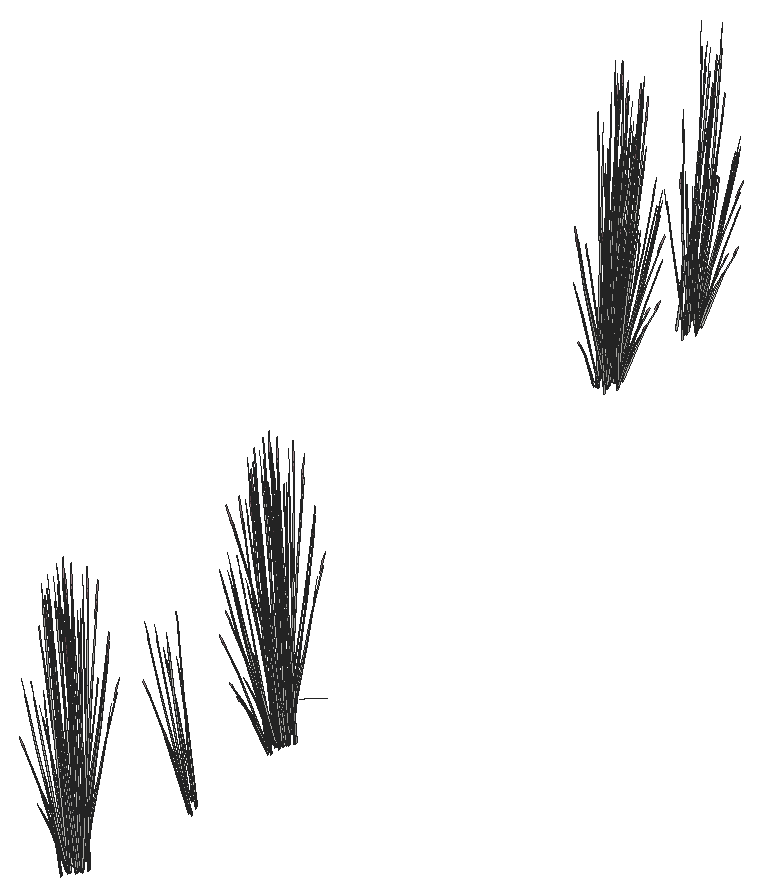
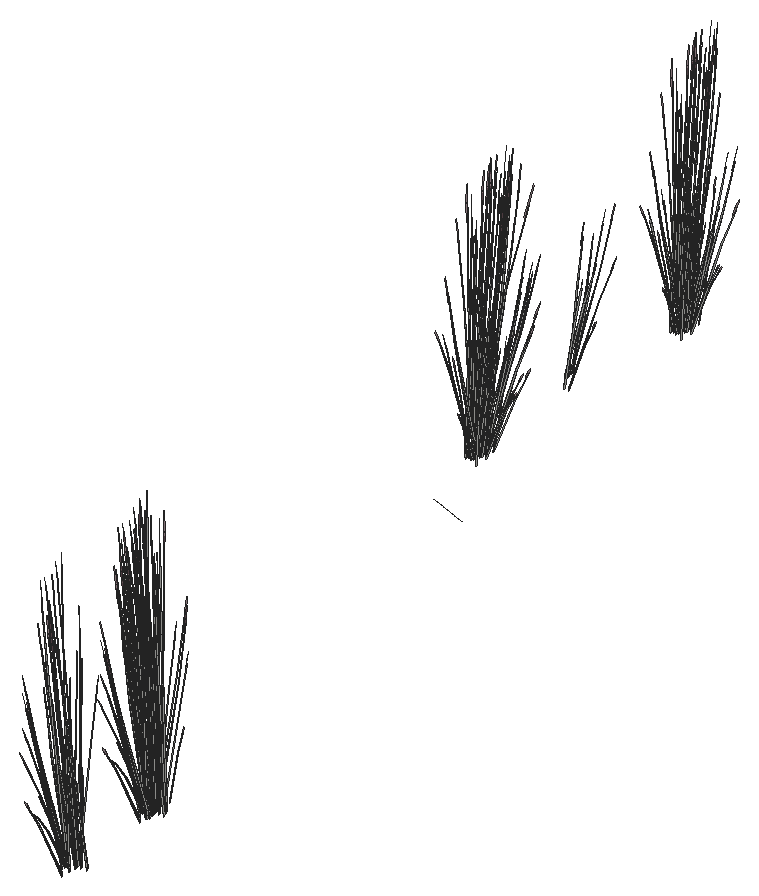
# SketchUp Ruby script. Lengths in inches.
U = 1.inch
M = Sketchup.active_model
def pt(a) = Geom::Point3d.new(a.map { |v| v * U })
def face(e, loops, mat)
  f = e.add_face(loops[0].map { |a| pt(a) })
  loops[1..].each { |l| e.add_face(l.map { |a| pt(a) }).erase! }
  f.material = f.back_material = mat if mat
  f
end
# faces: each face lists its corners as indices into pts; further lists are holes
def faces(e, pts, list, mat = nil) = list.each { |f| face(e, (f[0].is_a?(Array) ? f : [f]).map { |l| l.map { |i| pts[i] } }, mat) }
# xy, xz, yz: faces in a plane at the given z, y or x. An outline is a flat list of corners, or four numbers for a rectangle; further outlines are holes
def ring(l) = l.size == 4 ? [[l[0], l[1]], [l[2], l[1]], [l[2], l[3]], [l[0], l[3]]] : l.each_slice(2).to_a
def flat(e, list, mat, &to3) = list.each { |f| face(e, (f[0].is_a?(Array) ? f : [f]).map { |l| ring(l).map { |u, v| to3.(u, v) } }, mat) }
def xy(e, z, list, mat = nil) = flat(e, list, mat) { |x, y| [x, y, z] }
def xz(e, y, list, mat = nil) = flat(e, list, mat) { |x, z| [x, y, z] }
def yz(e, x, list, mat = nil) = flat(e, list, mat) { |y, z| [x, y, z] }
def lines(e, pts, list) = list.each { |a, b| e.add_line(pt(pts[a]), pt(pts[b])) }
# prism: a flat outline (further loops are holes) pulled along v
def prism(e, loops, v, mat = nil)
  f = face(e, loops, mat); d = Geom::Vector3d.new(v.map { |x| x * U })
  f.pushpull(f.normal.samedirection?(d) ? d.length : -d.length)
end
def box(e, o, s, mat = nil) = prism(e, [[o, [o[0] + s[0], o[1], o[2]], [o[0] + s[0], o[1] + s[1], o[2]], [o[0], o[1] + s[1], o[2]]]], [0, 0, s[2]], mat)
def at(x, y, z, deg = 0) = Geom::Transformation.translation(pt([x, y, z])) * Geom::Transformation.rotation(ORIGIN, Z_AXIS, deg.degrees)
def axes(o, x, y, z) = Geom::Transformation.new([*x, 0, *y, 0, *z, 0, *pt(o).to_a, 1])
def part(name) = M.definitions.add(name)
# library, detail: a bought-in or finely detailed component or shape, given as its bounding box
def library(name, o, s) = part(name).tap { |d| box(d.entities, o, s) }
def detail(e, o, s) = box(e.add_group.entities, o, s)
def put(e, d, t, mat = nil) = e.add_instance(d, t).tap { |i| i.material = mat if mat }
def group(e, t, mat = nil) = e.add_group.tap { |g| g.transformation = t; g.material = mat if mat }.entities
root = M.entities
M.materials.add("LightPink_Translucent").color = [144, 107, 117]
M.materials["LightPink_Translucent"].alpha = 0.75
c1 = part("blade")
p = [[2.15,0.21,22],[0,0.17,0],[0.09,0.45,0],[2.18,0.31,22],[2.29,0.31,22],[0.38,0.45,0],
  [2.48,0.24,33],[2.49,0.24,33],[2.48,0.22,33]]
faces(c1.entities,p,[[0,1,2,3],[4,5,2,3],[6,3,4,7],[8,0,3,6]])
c2 = part("seeds")
p = [[0.3,-0.1,1.38],[-0.01,-0.03,1.59],[-0.01,-0.03,0.03],[0.14,-0.07,-0.07],[0.29,-0.03,3],[0.15,0.01,3.11]]
faces(c2.entities,p,[[0,1,2,3],[1,0,4,5]],"LightPink_Translucent")
c3 = part("blade with seeds")
put(c3.entities,c1,at(0,0,0))
put(c3.entities,c2,axes([2.4,0.25,30.99],[1.5799,-0.05474,1.17369],[-0.12525,1.92788,0.29478],[-0.07173,-0.02425,1.56792]))
p = [[428.41,225.85,0],[423,225.85,-2]]
lines(root,p,[[0,1]])
put(root,c3,axes([402.14,327.82,-0.11],[-0.47029,-0.00441,-0.0428],[0,-0.61671,0.42951],[-0.01478,0.14039,1.36183]))
put(root,c3,axes([401.22,325.96,0.13],[-0.40434,0.14646,0.15172],[-0.09984,-0.54504,0.30174],[0.03606,0.07941,1.3795]))
put(root,c3,axes([399.88,348.72,-0.12],[0.39505,-0.18722,-0.1651],[0.13882,0.53931,0.00007],[0.04361,-0.02069,1.49552]))
put(root,c3,axes([400.8,323.92,0.38],[0.04827,0.32177,0.9878],[-0.26778,-0.17821,0.72577],[0.02882,-0.16476,0.21757]))
put(root,c3,axes([400.56,326.76,0.03],[-0.312,0.50076,0.39349],[-0.37066,-0.44204,0.15441],[0.07522,-0.04998,1.36617]))
put(root,c3,axes([401.09,327.55,-0.1],[0.26266,0.35642,0],[-0.26266,0.35642,0],[0,0,1.45569]))
put(root,c3,axes([401.08,327.13,0.34],[0.18257,-0.49721,0.38476],[0.37935,0.23929,-0.18517],[0,0.11462,1.23533]))
put(root,c3,axes([400.93,328.86,-0.1],[0.37935,0.24773,0],[-0.18257,0.51475,0],[0,0,1.5046]))
put(root,c3,axes([399.89,347.11,-0.1],[0.22605,0.46315,-0.38476],[-0.34239,0.32614,0.18517],[0.07315,0.05731,1.23533]))
put(root,c3,axes([400.39,329.51,2.03],[0.3699,0.13833,-0.43945],[-0.12679,0.47426,-0.34039],[0.03392,0.19095,0.84085]))
put(root,c3,axes([400.47,345.48,1.89],[0.2546,-0.29052,-0.30456],[0.24101,0.33173,0.39319],[0.03667,-0.16855,0.75234]))
put(root,c3,axes([400.96,327.01,0.05],[-0.4756,-0.11626,0.42311],[0.09679,-0.6566,0.16603],[0.0695,0.0634,1.46899]))
put(root,c3,axes([402.04,327.91,-0.26],[-0.26266,0.34428,-0.26641],[-0.26266,-0.34428,0.26641],[0,0.11089,1.19518]))
put(root,c3,axes([400.53,349.22,0.38],[-0.21187,-0.15866,0.9878],[0.27357,-0.16121,0.72577],[0.07379,0.13656,0.21757]))
put(root,c3,axes([399.77,349.05,0.23],[0.00664,-0.18292,1.22981],[0.31732,-0.20432,-0.26449],[0.09796,0.21893,0.52581]))
put(root,c3,axes([399.39,346.45,-0.23],[0.25345,-0.41475,-0.53624],[0.31485,0.37608,-0.14074],[0.10156,-0.10346,1.18365]))
put(root,c3,axes([401.29,327.84,-0.2],[0.13798,0.50522,-0.59522],[-0.39745,0.18195,-0.15622],[0.01525,0.17108,1.31385]))
put(root,c3,axes([401.1,327.3,-0.1],[0.42099,0,0],[0,0.57126,0],[0,0,1.5343]))
put(root,c3,axes([400.69,326.67,0.34],[-0.22605,-0.46315,0.38476],[0.34239,-0.32614,-0.18517],[0.07315,0.05731,1.23533]))
put(root,c3,axes([400.28,326.78,0.29],[-0.04385,-0.62963,-0.25022],[0.45669,-0.03807,-0.43002],[0.08042,-0.08387,1.37348]))
put(root,c3,axes([401.24,327.24,0.25],[0.35059,-0.16092,0.12452],[0.12277,0.45952,-0.35559],[0,0.10113,1.09]))
put(root,c3,axes([401.375,325.47,2.03],[-0.26937,-0.37076,-0.43945],[0.28456,-0.3247,-0.34039],[0.04099,-0.18838,0.84085]))
put(root,c3,axes([400.51,346.09,-0.26],[0.08839,0.48081,-0.26641],[-0.35106,0.13653,0.26641],[0.07077,0.05545,1.19518]))
put(root,c3,axes([401.17,347.65,0.04],[0.47052,0,0],[0,0.61671,-0.44382],[0,0.14046,1.40792]))
put(root,c3,axes([401.125,327.28,0.29],[0.42377,0.26329,-0.25022],[-0.20405,0.55571,-0.43002],[0.01332,0.13644,1.37348]))
put(root,c3,axes([399.65,346.85,0.29],[0.37992,-0.36634,-0.25022],[0.25264,0.51764,-0.43002],[0.09374,0.05257,1.37348]))
put(root,c3,axes([400.5625,349.9375,0.29],[-0.2413,-0.01731,0.90352],[0.15935,-0.36755,0.49885],[0.09532,0.13058,0.70873]))
put(root,c3,axes([400.22,325.39,-0.26],[0.35106,0.13653,-0.26641],[-0.08839,0.48081,0.26641],[0.07077,-0.05545,1.19518]))
put(root,c3,axes([401.2,324.81,0.23],[-0.10696,0.11169,1.22981],[-0.32033,-0.19549,-0.26449],[0.05938,-0.24312,0.52581]))
put(root,c3,axes([402.04,327.41,0.13],[0,-0.5518,0.427],[0.42099,0,0],[0,0.12568,1.35453]))
put(root,c3,axes([402.22,327.92,-0.26],[0,0.5518,-0.427],[-0.42099,0,0],[0,0.12568,1.35453]))
put(root,c3,axes([400.14,325.17,-0.26],[0.35217,-0.2759,-0.427],[0.2105,0.49473,0],[0.08021,-0.06284,1.35453]))
put(root,c3,axes([400.84,326.54,0.25],[0.07259,-0.49245,0.12452],[0.35466,0.08548,-0.35559],[0.06454,0.05057,1.09]))
put(root,c3,axes([398.6875,346.53,-0.63],[-0.37038,0.22092,1.10879],[-0.11789,-0.63387,0.43083],[0.22743,0.01055,1.26112]))
put(root,c3,axes([401.35,325.68,0.13],[-0.35217,-0.2759,0.427],[0.2105,-0.49473,0],[0.08021,0.06284,1.35453]))
put(root,c3,axes([401.46,325.64,2.28],[0.00979,-0.51041,-0.61099],[0.4123,0.03428,0.07373],[0.04351,-0.21623,0.8643]))
put(root,c3,axes([400.05,349.43,2.03],[0.37131,-0.13117,-0.43945],[0.06495,0.49674,-0.34039],[0.09973,0.14235,0.84085]))
put(root,c3,axes([401.04,328.5625,-0.12],[0.39505,-0.18722,-0.1651],[0.13882,0.53931,0.00007],[0.04361,-0.02069,1.49552]))
put(root,c3,axes([400.39,345.55,0.04],[0.23526,-0.55293,0],[0.3936,0.30836,-0.44382],[0.08964,0.07023,1.40792]))
put(root,c3,axes([400.78,345.31,-0.72],[-0.05632,-0.04347,1.51654],[-0.14467,-0.48565,-0.23168],[0.09759,-0.13179,0.25832]))
put(root,c3,axes([400.6,345.88,-0.26],[0.35217,0.2759,-0.427],[-0.2105,0.49473,0],[0.08021,0.06284,1.35453]))
put(root,c3,axes([400.59,349.8,-0.72],[0.02741,-0.07966,1.51654],[0.34514,-0.23462,-0.23168],[0.10464,0.12143,0.25832]))
put(root,c3,axes([400.77,346.47,2.03],[-0.09666,-0.50384,-0.43945],[0.36608,-0.08814,-0.34039],[0.10491,-0.13533,0.84085]))
put(root,c3,axes([401.05,326.96,-0.1],[0.22605,0.46315,-0.38476],[-0.34239,0.32614,0.18517],[0.07315,0.05731,1.23533]))
put(root,c3,axes([401.63,325.33,1.89],[0.2546,-0.29052,-0.30456],[0.24101,0.33173,0.39319],[0.03667,-0.16855,0.75234]))
put(root,c3,axes([400.09,346.9375,-0.23],[0.39143,0.09047,-0.53624],[-0.0826,0.55804,-0.14074],[0.11681,0.06762,1.18365]))
put(root,c3,axes([401.6875,329.0625,0.38],[-0.21187,-0.15866,0.9878],[0.27357,-0.16121,0.72577],[0.07379,0.13656,0.21757]))
put(root,c3,axes([400.94,328.89,0.23],[0.00664,-0.18292,1.22981],[0.31732,-0.20432,-0.26449],[0.09796,0.21893,0.52581]))
put(root,c3,axes([401.76,347.26,-0.06],[-0.23329,-0.35284,-0.05579],[0.2555,-0.3233,-0.25298],[0.0724,-0.02276,0.83441]))
put(root,c3,axes([400.56,326.3,-0.23],[0.25345,-0.41475,-0.53624],[0.31485,0.37608,-0.14074],[0.10156,-0.10346,1.18365]))
put(root,c3,axes([401.22,345.47,0.38],[-0.12533,0.28089,0.9878],[-0.10773,-0.37739,0.72577],[0.10352,-0.09457,0.21757]))
put(root,c3,axes([401.67,325.93,-0.26],[0.08839,0.48081,-0.26641],[-0.35106,0.13653,0.26641],[0.07077,0.05545,1.19518]))
put(root,c3,axes([402.33,327.5,0.04],[0.47052,0,0],[0,0.61671,-0.44382],[0,0.14046,1.40792]))
put(root,c3,axes([400.81,326.7,0.29],[0.37992,-0.36634,-0.25022],[0.25264,0.51764,-0.43002],[0.09374,0.05257,1.37348]))
put(root,c3,axes([401.72,329.78,0.29],[-0.2413,-0.01731,0.90352],[0.15935,-0.36755,0.49885],[0.09532,0.13058,0.70873]))
put(root,c3,axes([401.04,346.52,1.89],[0.32754,-0.07886,-0.30456],[0.08649,0.45081,0.39319],[0.09386,-0.12109,0.75234]))
put(root,c3,axes([400.78,346.68,2.28],[0.19655,-0.43539,-0.61099],[0.34443,0.30942,0.07373],[0.11736,-0.15774,0.8643]))
put(root,c3,axes([400.78,349.02,1.89],[0.2141,0.34548,-0.30456],[-0.24447,0.32704,0.39319],[0.12421,0.04976,0.75234]))
put(root,c3,axes([399.85,326.375,-0.63],[-0.37038,0.22092,1.10879],[-0.11789,-0.63387,0.43083],[0.22743,0.01055,1.26112]))
put(root,c3,axes([401.21,329.28,2.03],[0.37131,-0.13117,-0.43945],[0.06495,0.49674,-0.34039],[0.09973,0.14235,0.84085]))
put(root,c3,axes([401.55,325.39,0.04],[0.23526,-0.55293,0],[0.3936,0.30836,-0.44382],[0.08964,0.07023,1.40792]))
put(root,c3,axes([401.95,325.15,-0.72],[-0.05632,-0.04347,1.51654],[-0.14467,-0.48565,-0.23168],[0.09759,-0.13179,0.25832]))
put(root,c3,axes([401.77,325.73,-0.26],[0.35217,0.2759,-0.427],[-0.2105,0.49473,0],[0.08021,0.06284,1.35453]))
put(root,c3,axes([400.94,347.59,2.03],[0.10194,-0.50193,-0.43945],[0.34951,0.17204,-0.34039],[0.14072,-0.04602,0.84085]))
put(root,c3,axes([401.82,347.91,0.38],[-0.23249,0.0911,0.9878],[0.10944,-0.37648,0.72577],[0.12334,0.02576,0.21757]))
put(root,c3,axes([401.75,329.65,-0.72],[0.02741,-0.07966,1.51654],[0.34514,-0.23462,-0.23168],[0.10464,0.12143,0.25832]))
put(root,c3,axes([401.93,326.32,2.03],[-0.09666,-0.50384,-0.43945],[0.36608,-0.08814,-0.34039],[0.10491,-0.13533,0.84085]))
put(root,c3,axes([401.07,346.27,0.23],[-0.13443,-0.01634,1.22981],[-0.13772,-0.43844,-0.26449],[0.16514,-0.12403,0.52581]))
put(root,c3,axes([401.16,347.82,1.89],[0.31272,0.15393,-0.30456],[-0.09121,0.44909,0.39319],[0.1259,-0.04118,0.75234]))
put(root,c3,axes([401.25,326.78,-0.23],[0.39143,0.09047,-0.53624],[-0.0826,0.55804,-0.14074],[0.11681,0.06762,1.18365]))
put(root,c3,axes([402.92,327.11,-0.06],[-0.23329,-0.35284,-0.05579],[0.2555,-0.3233,-0.25298],[0.0724,-0.02276,0.83441]))
put(root,c3,axes([400.55,348.79,2.28],[0.37615,0.01329,-0.61099],[-0.02526,0.55946,0.07373],[0.15935,0.05904,0.8643]))
put(root,c3,axes([401.32,347.73,-0.3],[-0.24235,0.06622,1.21762],[-0.03858,-0.5271,0.0697],[0.16974,-0.07978,0.69287]))
put(root,c3,axes([402.38,325.32,0.38],[-0.12533,0.28089,0.9878],[-0.10773,-0.37739,0.72577],[0.10352,-0.09457,0.21757]))
put(root,c3,axes([401.58,347.39,-0.72],[-0.01967,-0.08377,1.51654],[0.1364,-0.49004,-0.23168],[0.13759,-0.00705,0.25832]))
put(root,c3,axes([400.875,347.77,2.28],[0.33065,-0.2437,-0.61099],[0.18427,0.50165,0.07373],[0.15976,-0.05699,0.8643]))
put(root,c3,axes([402.2,326.37,1.89],[0.32754,-0.07886,-0.30456],[0.08649,0.45081,0.39319],[0.09386,-0.12109,0.75234]))
put(root,c3,axes([401.94,326.52,2.28],[0.19655,-0.43539,-0.61099],[0.34443,0.30942,0.07373],[0.11736,-0.15774,0.8643]))
put(root,c3,axes([401.94,328.87,1.89],[0.2141,0.34548,-0.30456],[-0.24447,0.32704,0.39319],[0.12421,0.04976,0.75234]))
put(root,c3,axes([401.38,348.51,0.23],[-0.09062,-0.13571,1.22981],[0.11791,-0.44895,-0.26449],[0.18335,0.06082,0.52581]))
put(root,c3,axes([402.1,327.4375,2.03],[0.10194,-0.50193,-0.43945],[0.34951,0.17204,-0.34039],[0.14072,-0.04602,0.84085]))
put(root,c3,axes([402.98,327.76,0.38],[-0.23249,0.0911,0.9878],[0.10944,-0.37648,0.72577],[0.12334,0.02576,0.21757]))
put(root,c3,axes([402.23,326.12,0.23],[-0.13443,-0.01634,1.22981],[-0.13772,-0.43844,-0.26449],[0.16514,-0.12403,0.52581]))
put(root,c3,axes([402.32,327.67,1.89],[0.31272,0.15393,-0.30456],[-0.09121,0.44909,0.39319],[0.1259,-0.04118,0.75234]))
put(root,c3,axes([401.71,328.64,2.28],[0.37615,0.01329,-0.61099],[-0.02526,0.55946,0.07373],[0.15935,0.05904,0.8643]))
put(root,c3,axes([402.48,327.58,-0.3],[-0.24235,0.06622,1.21762],[-0.03858,-0.5271,0.0697],[0.16974,-0.07978,0.69287]))
put(root,c3,axes([402.74,327.23,-0.72],[-0.01967,-0.08377,1.51654],[0.1364,-0.49004,-0.23168],[0.13759,-0.00705,0.25832]))
put(root,c3,axes([402.04,327.62,2.28],[0.33065,-0.2437,-0.61099],[0.18427,0.50165,0.07373],[0.15976,-0.05699,0.8643]))
put(root,c3,axes([402.55,328.36,0.23],[-0.09062,-0.13571,1.22981],[0.11791,-0.44895,-0.26449],[0.18335,0.06082,0.52581]))
put(root,c3,axes([430.46,162.27,0.23],[0.13077,0.0453,1.22981],[0.08428,0.46268,-0.26449],[-0.17763,0.08661,0.52581]))
put(root,c3,axes([430.46,211.47,0.23],[0.13077,0.0453,1.22981],[0.08428,0.46268,-0.26449],[-0.17763,0.08661,0.52581]))
put(root,c3,axes([431.62,160.79,0.875],[0.10696,-0.07982,1.52275],[0.03688,0.55733,0.11917],[-0.23167,0.07395,0.54424]))
put(root,c3,axes([431.62,209.99,0.875],[0.10696,-0.07982,1.52275],[0.03688,0.55733,0.11917],[-0.23167,0.07395,0.54424]))
put(root,c3,axes([431.27,159.9,2.28],[-0.37615,-0.01329,-0.61099],[0.02526,-0.55946,0.07373],[-0.15935,-0.05904,0.8643]))
put(root,c3,axes([431.27,209.09,2.28],[-0.37615,-0.01329,-0.61099],[0.02526,-0.55946,0.07373],[-0.15935,-0.05904,0.8643]))
put(root,c3,axes([430.97,160.03,0.23],[0.07347,0.15363,1.22981],[-0.16929,0.41759,-0.26449],[-0.17383,-0.09981,0.52581]))
put(root,c3,axes([430.97,209.23,0.23],[0.07347,0.15363,1.22981],[-0.16929,0.41759,-0.26449],[-0.17383,-0.09981,0.52581]))
put(root,c3,axes([430.67,160.87,1.89],[-0.31272,-0.15393,-0.30456],[0.09121,-0.44909,0.39319],[-0.1259,0.04118,0.75234]))
put(root,c3,axes([430.88,161.1,2.03],[-0.10194,0.50193,-0.43945],[-0.34951,-0.17204,-0.34039],[-0.14072,0.04602,0.84085]))
put(root,c3,axes([430.88,210.29,2.03],[-0.10194,0.50193,-0.43945],[-0.34951,-0.17204,-0.34039],[-0.14072,0.04602,0.84085]))
put(root,c3,axes([431.15,160.01,2.03],[-0.27323,0.36552,-0.43945],[-0.23929,-0.38612,-0.34039],[-0.13882,-0.05561,0.84085]))
put(root,c3,axes([431.15,209.21,2.03],[-0.27323,0.36552,-0.43945],[-0.23929,-0.38612,-0.34039],[-0.13882,-0.05561,0.84085]))
put(root,c3,axes([430.71,161.06,-0.72],[0.00954,0.08696,1.51654],[-0.19238,0.45414,-0.23168],[-0.13665,-0.02289,0.25832]))
put(root,c3,axes([430.71,210.26,-0.72],[0.00954,0.08696,1.51654],[-0.19238,0.45414,-0.23168],[-0.13665,-0.02289,0.25832]))
put(root,c3,axes([430.19,163.24,0.38],[0.15682,-0.25009,0.9878],[0.06188,0.39591,0.72577],[-0.11333,0.07089,0.21757]))
put(root,c3,axes([430.19,212.4375,0.38],[0.15682,-0.25009,0.9878],[0.06188,0.39591,0.72577],[-0.11333,0.07089,0.21757]))
put(root,c3,axes([430.78,162.16,1.89],[-0.32754,0.07886,-0.30456],[-0.08649,-0.45081,0.39319],[-0.09386,0.12109,0.75234]))
put(root,c3,axes([430.6,163.5,-0.72],[0.05047,0.05513,1.51654],[0.08558,0.51079,-0.23168],[-0.11187,0.10892,0.25832]))
put(root,c3,axes([430.6,212.7,-0.72],[0.05047,0.05513,1.51654],[0.08558,0.51079,-0.23168],[-0.11187,0.10892,0.25832]))
put(root,c3,axes([430.53,160.5,0.38],[0.24023,-0.03948,0.9878],[-0.15239,0.3479,0.72577],[-0.11872,-0.05219,0.21757]))
put(root,c3,axes([430.53,209.69,0.38],[0.24023,-0.03948,0.9878],[-0.15239,0.3479,0.72577],[-0.11872,-0.05219,0.21757]))
put(root,c3,axes([431.05,162.21,2.03],[0.09666,0.50384,-0.43945],[-0.36608,0.08814,-0.34039],[-0.10491,0.13533,0.84085]))
put(root,c3,axes([431.05,211.41,2.03],[0.09666,0.50384,-0.43945],[-0.36608,0.08814,-0.34039],[-0.10491,0.13533,0.84085]))
put(root,c3,axes([431.97,161.85,-0.23],[-0.39143,-0.09047,-0.53624],[0.0826,-0.55804,-0.14074],[-0.11681,-0.06762,1.18365]))
put(root,c3,axes([431.97,211.05,-0.23],[-0.39143,-0.09047,-0.53624],[0.0826,-0.55804,-0.14074],[-0.11681,-0.06762,1.18365]))
put(root,c3,axes([431.93,208.43,2.28],[-0.32086,-0.26671,-0.61099],[0.22803,-0.46737,0.07373],[-0.11625,-0.15925,0.8643]))
put(root,c3,axes([431.78,208.45,2.03],[-0.37131,0.13117,-0.43945],[-0.06495,-0.49674,-0.34039],[-0.09973,-0.14235,0.84085]))
put(root,c3,axes([431.45,162.91,-0.26],[-0.35217,-0.2759,-0.427],[0.2105,-0.49473,0],[-0.08021,-0.06284,1.35453]))
put(root,c3,axes([431.45,212.11,-0.26],[-0.35217,-0.2759,-0.427],[0.2105,-0.49473,0],[-0.08021,-0.06284,1.35453]))
put(root,c3,axes([431.3,208,-0.72],[-0.03645,0.07269,1.51654],[-0.36835,0.15672,-0.23168],[-0.08898,-0.14257,0.25832]))
put(root,c3,axes([431.67,163.24,0.04],[-0.23526,0.55293,0],[-0.3936,-0.30836,-0.44382],[-0.08964,-0.07023,1.40792]))
put(root,c3,axes([431.67,212.4375,0.04],[-0.23526,0.55293,0],[-0.3936,-0.30836,-0.44382],[-0.08964,-0.07023,1.40792]))
put(root,c3,axes([431.24,164.04,0.23],[0.11874,-0.08705,1.22981],[0.29317,0.26247,-0.26449],[-0.08726,0.22711,0.52581]))
put(root,c3,axes([431.24,213.24,0.23],[0.11874,-0.08705,1.22981],[0.29317,0.26247,-0.26449],[-0.08726,0.22711,0.52581]))
put(root,c3,axes([431.07,159.08,-0.17],[-0.10855,0.45057,-0.03348],[-0.33409,-0.1386,-0.15179],[-0.05073,-0.0737,0.50065]))
put(root,c3,axes([431.07,208.28,-0.17],[-0.10855,0.45057,-0.03348],[-0.33409,-0.1386,-0.15179],[-0.05073,-0.0737,0.50065]))
put(root,c3,axes([431.57,207.71,0.23],[-0.02279,0.18051,1.22981],[-0.33311,0.15111,-0.26449],[-0.07787,-0.23331,0.52581]))
put(root,c3,axes([432.41,161.94,0.29],[-0.37992,0.36634,-0.25022],[-0.25264,-0.51764,-0.43002],[-0.09374,-0.05257,1.37348]))
put(root,c3,axes([432.41,211.13,0.29],[-0.37992,0.36634,-0.25022],[-0.25264,-0.51764,-0.43002],[-0.09374,-0.05257,1.37348]))
put(root,c3,axes([430.89,161.14,0.04],[-0.47052,0,0],[0,-0.61671,-0.44382],[0,-0.14046,1.40792]))
put(root,c3,axes([430.89,210.33,0.04],[-0.47052,0,0],[0,-0.61671,-0.44382],[0,-0.14046,1.40792]))
put(root,c3,axes([431.55,162.7,-0.26],[-0.08839,-0.48081,-0.26641],[0.35106,-0.13653,0.26641],[-0.07077,-0.05545,1.19518]))
put(root,c3,axes([431.55,211.9,-0.26],[-0.08839,-0.48081,-0.26641],[0.35106,-0.13653,0.26641],[-0.07077,-0.05545,1.19518]))
put(root,c3,axes([431.36,163.21,1.89],[-0.2546,0.29052,-0.30456],[-0.24101,-0.33173,0.39319],[-0.03667,0.16855,0.75234]))
put(root,c3,axes([432.66,162.34,-0.23],[-0.25345,0.41475,-0.53624],[-0.31485,-0.37608,-0.14074],[-0.10156,0.10346,1.18365]))
put(root,c3,axes([432.66,211.53,-0.23],[-0.25345,0.41475,-0.53624],[-0.31485,-0.37608,-0.14074],[-0.10156,0.10346,1.18365]))
put(root,c3,axes([431.25,160.97,0],[-0.35001,0.46392,0.2645],[-0.35022,-0.45904,-0.31383],[-0.01222,-0.13174,1.41801]))
put(root,c3,axes([431.25,210.17,0],[-0.35001,0.46392,0.2645],[-0.35022,-0.45904,-0.31383],[-0.01222,-0.13174,1.41801]))
put(root,c3,axes([432.69,211.45,0.86],[0.32517,0.22251,1.30084],[-0.31856,0.47936,0.51441],[-0.14269,-0.28411,1.09053]))
put(root,c3,axes([431.45,207.42,0.38],[0.19628,0.19205,0.9878],[-0.28586,0.11545,0.72577],[-0.06116,-0.1476,0.21757]))
put(root,c3,axes([432.84,162.1,0.12],[-0.36743,-0.44413,-0.21665],[0.30918,-0.49872,0.47412],[-0.09894,0.05195,1.44665]))
put(root,c3,axes([432.84,211.3,0.12],[-0.36743,-0.44413,-0.21665],[0.30918,-0.49872,0.47412],[-0.09894,0.05195,1.44665]))
put(root,c3,axes([432.17,161.68,-0.1],[-0.22605,-0.46315,-0.38476],[0.34239,-0.32614,0.18517],[-0.07315,-0.05731,1.23533]))
put(root,c3,axes([432.17,210.87,-0.1],[-0.22605,-0.46315,-0.38476],[0.34239,-0.32614,0.18517],[-0.07315,-0.05731,1.23533]))
put(root,c3,axes([431.53,162.9,2.59],[-0.00979,0.51041,-0.6782],[-0.4123,-0.03428,0.08184],[-0.04351,0.21623,0.95938]))
put(root,c3,axes([431.53,212.09,2.59],[-0.00979,0.51041,-0.6782],[-0.4123,-0.03428,0.08184],[-0.04351,0.21623,0.95938]))
put(root,c3,axes([431.52,164.33,0.38],[-0.00974,-0.3281,0.9878],[0.24334,0.23402,0.72577],[-0.04786,0.15639,0.21757]))
put(root,c3,axes([431.52,213.53,0.38],[-0.00974,-0.3281,0.9878],[0.24334,0.23402,0.72577],[-0.04786,0.15639,0.21757]))
put(root,c3,axes([432.65,162.01,-0.1],[-0.40861,0.03406,-0.38476],[-0.03695,-0.56543,0.18517],[-0.07315,0.05731,1.23533]))
put(root,c3,axes([432.65,211.2,-0.1],[-0.40861,0.03406,-0.38476],[-0.03695,-0.56543,0.18517],[-0.07315,0.05731,1.23533]))
put(root,c3,axes([431.87,162.95,0.13],[0.35217,0.2759,0.427],[-0.2105,0.49473,0],[-0.08021,-0.06284,1.35453]))
put(root,c3,axes([431.87,212.15,0.13],[0.35217,0.2759,0.427],[-0.2105,0.49473,0],[-0.08021,-0.06284,1.35453]))
put(root,c3,axes([431.39,163.62,0.89],[0.00827,-0.28486,1.32737],[0.37184,0.15046,0.18343],[-0.03222,0.30359,0.62678]))
put(root,c3,axes([431.39,212.8125,0.89],[0.00827,-0.28486,1.32737],[0.37184,0.15046,0.18343],[-0.03222,0.30359,0.62678]))
put(root,c3,axes([433.92,187.37,0.23],[0.13077,0.0453,1.22981],[0.08428,0.46268,-0.26449],[-0.17763,0.08661,0.52581]))
put(root,c3,axes([432.2,161.94,0.1],[0.09973,-0.65385,-0.20149],[0.47288,0.11397,0.44093],[-0.08263,-0.0903,1.34539]))
put(root,c3,axes([432.2,211.14,0.1],[0.09973,-0.65385,-0.20149],[0.47288,0.11397,0.44093],[-0.08263,-0.0903,1.34539]))
put(root,c3,axes([432.375,162.1,0.25],[-0.07259,0.49245,0.12452],[-0.35466,-0.08548,-0.35559],[-0.06454,-0.05057,1.09]))
put(root,c3,axes([432.375,211.29,0.25],[-0.07259,0.49245,0.12452],[-0.35466,-0.08548,-0.35559],[-0.06454,-0.05057,1.09]))
put(root,c3,axes([435.07,185.89,0.875],[0.10696,-0.07982,1.52275],[0.03688,0.55733,0.11917],[-0.23167,0.07395,0.54424]))
put(root,c3,axes([433.08,163.47,-0.26],[-0.35217,0.2759,-0.427],[-0.2105,-0.49473,0],[-0.08021,0.06284,1.35453]))
put(root,c3,axes([433.08,212.66,-0.26],[-0.35217,0.2759,-0.427],[-0.2105,-0.49473,0],[-0.08021,0.06284,1.35453]))
put(root,c3,axes([430.99,209.91,-0.26],[0,-0.5518,-0.427],[0.42099,0,0],[0,-0.12568,1.35453]))
put(root,c3,axes([431.17,161.23,0.13],[0,0.5518,0.427],[-0.42099,0,0],[0,-0.12568,1.35453]))
put(root,c3,axes([431.17,210.43,0.13],[0,0.5518,0.427],[-0.42099,0,0],[0,-0.12568,1.35453]))
put(root,c3,axes([433.1,163.32,-0.11],[-0.23233,-0.55486,-0.04422],[0.3936,-0.30836,0.44382],[-0.09699,0.05283,1.40722]))
put(root,c3,axes([433.1,212.52,-0.11],[-0.23233,-0.55486,-0.04422],[0.3936,-0.30836,0.44382],[-0.09699,0.05283,1.40722]))
put(root,c3,axes([431.61,163.07,2.3],[0.26937,0.37076,-0.48779],[-0.28456,0.3247,-0.37783],[-0.04099,0.18838,0.93334]))
put(root,c3,axes([431.61,212.26,2.3],[0.26937,0.37076,-0.48779],[-0.28456,0.3247,-0.37783],[-0.04099,0.18838,0.93334]))
put(root,c3,axes([433,163.25,-0.26],[-0.35106,-0.13653,-0.26641],[0.08839,-0.48081,0.26641],[-0.07077,0.05545,1.19518]))
put(root,c3,axes([433,212.44,-0.26],[-0.35106,-0.13653,-0.26641],[0.08839,-0.48081,0.26641],[-0.07077,0.05545,1.19518]))
put(root,c3,axes([432.09,161.36,0.29],[-0.42377,-0.26329,-0.25022],[0.20405,-0.55571,-0.43002],[-0.01332,-0.13644,1.37348]))
put(root,c3,axes([432.09,210.55,0.29],[-0.42377,-0.26329,-0.25022],[0.20405,-0.55571,-0.43002],[-0.01332,-0.13644,1.37348]))
put(root,c3,axes([433.2,161.19,0.44],[-0.01028,-0.51954,1.21494],[0.46521,0.13467,0.51441],[-0.11003,0.28429,1.14681]))
put(root,c3,axes([433.2,210.39,0.44],[-0.01028,-0.51954,1.21494],[0.46521,0.13467,0.51441],[-0.11003,0.28429,1.14681]))
put(root,c3,axes([434.73,185,2.28],[-0.37615,-0.01329,-0.61099],[0.02526,-0.55946,0.07373],[-0.15935,-0.05904,0.8643]))
put(root,c3,axes([434.42,185.13,0.23],[0.07347,0.15363,1.22981],[-0.16929,0.41759,-0.26449],[-0.17383,-0.09981,0.52581]))
put(root,c3,axes([434.12,185.97,1.89],[-0.31272,-0.15393,-0.30456],[0.09121,-0.44909,0.39319],[-0.1259,0.04118,0.75234]))
put(root,c3,axes([431.32,163.625,0.43],[0.34184,-0.09771,0.05596],[0.07859,0.39367,-0.74222],[-0.02167,0.19928,0.6653]))
put(root,c3,axes([431.32,212.82,0.43],[0.34184,-0.09771,0.05596],[0.07859,0.39367,-0.74222],[-0.02167,0.19928,0.6653]))
put(root,c3,axes([432.9375,161.85,0.29],[0.04385,0.62963,-0.25022],[-0.45669,0.03807,-0.43002],[-0.08042,0.08387,1.37348]))
put(root,c3,axes([432.9375,211.05,0.29],[0.04385,0.62963,-0.25022],[-0.45669,0.03807,-0.43002],[-0.08042,0.08387,1.37348]))
put(root,c3,axes([431.9,209.99,-0.2],[-0.15453,-0.56584,-0.60058],[0.44514,-0.20379,-0.15763],[-0.01708,-0.19161,1.32568]))
put(root,c3,axes([432.6,208.22,2.03],[-0.3699,-0.13833,-0.43945],[0.12679,-0.47426,-0.34039],[-0.03392,-0.19095,0.84085]))
put(root,c3,axes([434.34,186.19,2.03],[-0.10194,0.50193,-0.43945],[-0.34951,-0.17204,-0.34039],[-0.14072,0.04602,0.84085]))
put(root,c3,axes([431.17,160.73,-0.26],[0.26266,-0.34428,-0.26641],[0.26266,0.34428,0.26641],[0,-0.11089,1.19518]))
put(root,c3,axes([431.17,209.93,-0.26],[0.26266,-0.34428,-0.26641],[0.26266,0.34428,0.26641],[0,-0.11089,1.19518]))
put(root,c3,axes([432.36,207.7,-0.17],[-0.26003,0.31656,-0.03348],[-0.23826,-0.3467,-0.15179],[-0.01677,-0.09824,0.50065]))
put(root,c3,axes([434.6,185.11,2.03],[-0.27323,0.36552,-0.43945],[-0.23929,-0.38612,-0.34039],[-0.13882,-0.05561,0.84085]))
put(root,c3,axes([434.16,186.16,-0.72],[0.00954,0.08696,1.51654],[-0.19238,0.45414,-0.23168],[-0.13665,-0.02289,0.25832]))
put(root,c3,axes([432.26,161.625,0.03],[0.4756,0.11626,0.39349],[-0.09679,0.6566,0.15441],[-0.0695,-0.0634,1.36617]))
put(root,c3,axes([432.26,210.82,0.03],[0.4756,0.11626,0.39349],[-0.09679,0.6566,0.15441],[-0.0695,-0.0634,1.36617]))
put(root,c3,axes([432.13,161.51,0.34],[-0.18257,0.49721,0.38476],[-0.37935,-0.23929,-0.18517],[0,-0.11462,1.23533]))
put(root,c3,axes([432.13,210.7,0.34],[-0.18257,0.49721,0.38476],[-0.37935,-0.23929,-0.18517],[0,-0.11462,1.23533]))
